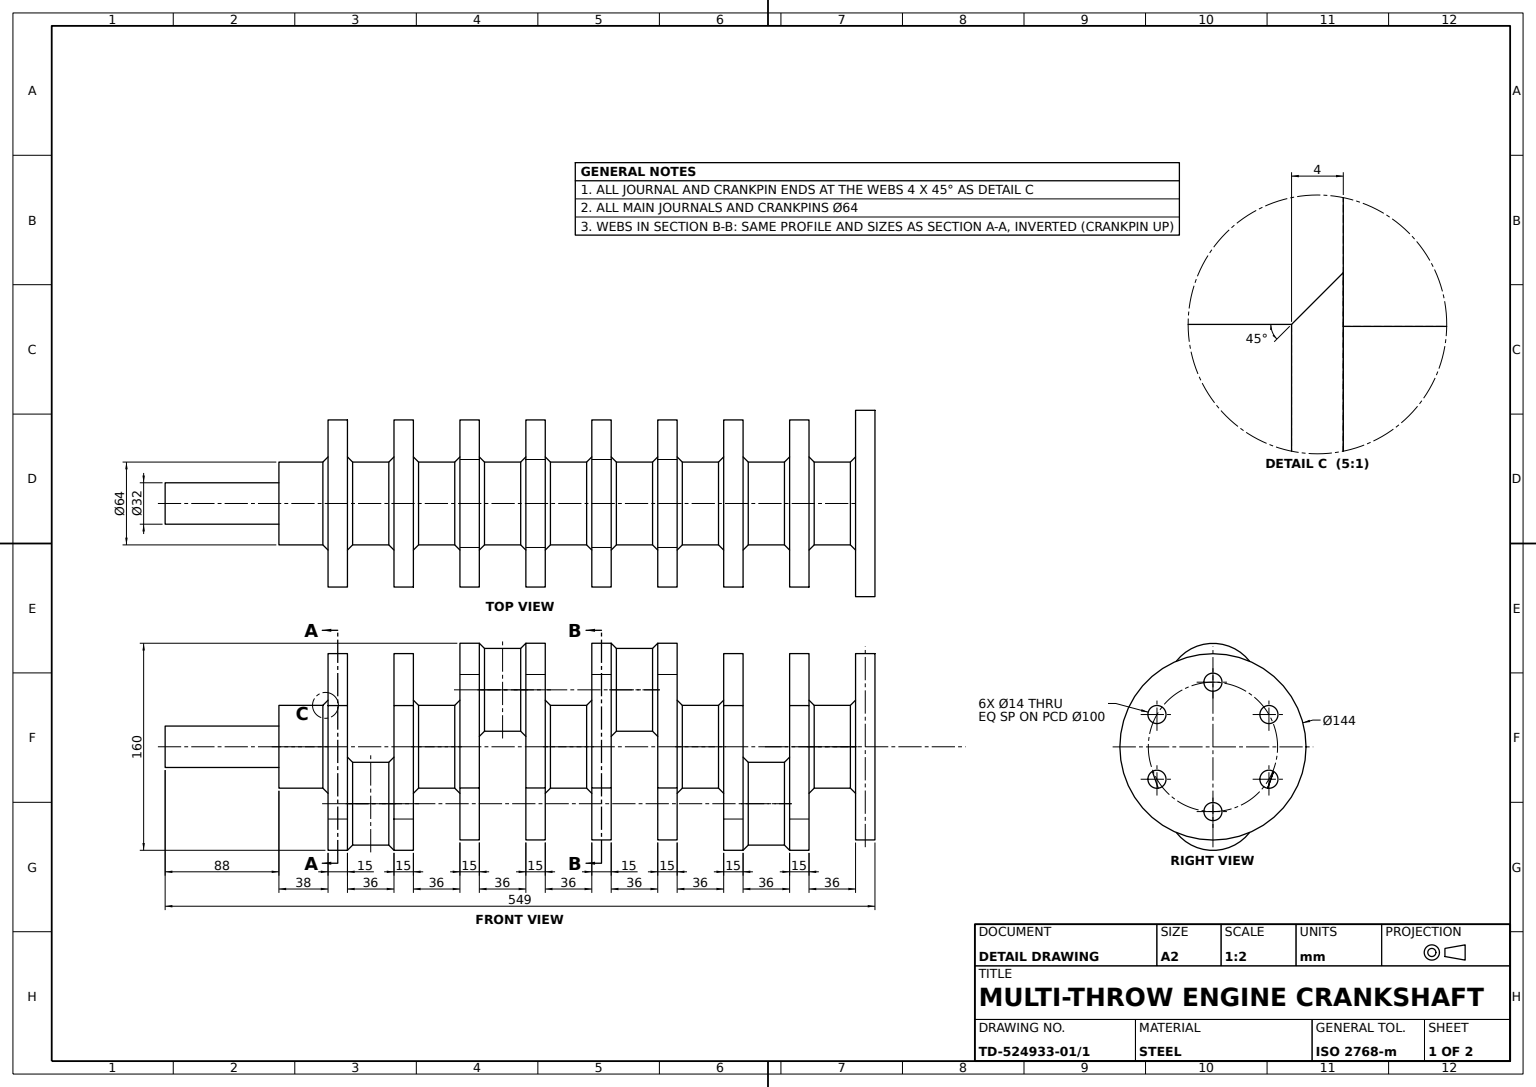
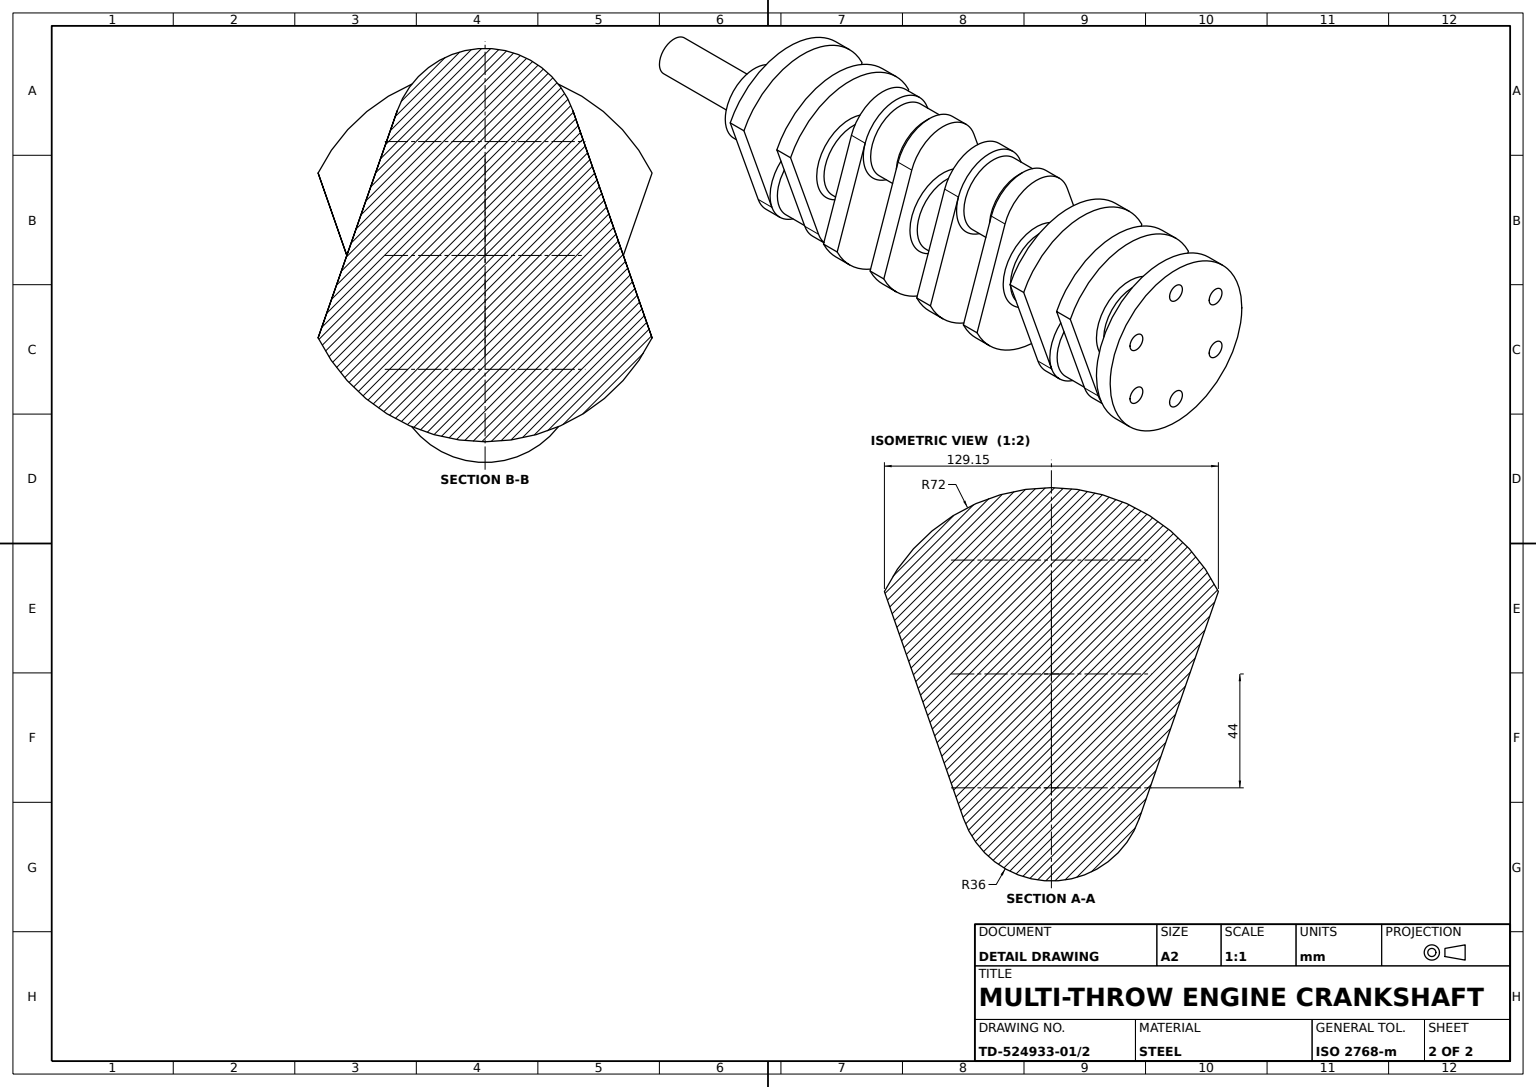
solid
v1 (32,-44,-85)
v2 (36,-44,-89)
e1 v1 v2 LINE
v3 (-36,-44,-89)
e2 v3 v2 CIRCLE(AX(P(0,-44,-89),D(0,0,-1),D(-1,0,0)),36)
v4 (-32,-44,-85)
e3 v4 v3 LINE
e4 v1 v4 CIRCLE(AX(P(0,-44,-85),D(0,0,1),D(-1,0,0)),32)
face CONE(AX(P(0,-44,-89),D(0,0,-1),D(-1,0,0)),36,0.785398163) [e1 -e2 -e3 -e4]
v5 (33.992546,55.853557,-206)
v6 (33.992546,55.853557,-191)
e5 v5 v6 LINE
v7 (-33.992546,55.853557,-206)
e6 v7 v5 CIRCLE(AX(P(0,44,-206),D(0,0,-1),D(-1,0,0)),36)
v8 (-33.992546,55.853557,-191)
e7 v7 v8 LINE
e8 v8 v6 CIRCLE(AX(P(0,44,-191),D(0,0,-1),D(-1,0,0)),36)
face CYL(AX(P(0,44,-206),D(0,0,1),D(1,0,0)),36) [-e5 -e6 e7 e8]
v9 (32,-44,-363)
v10 (-32,-44,-363)
e9 v9 v10 CIRCLE(AX(P(0,-44,-363),D(0,0,-1),D(-1,0,0)),32)
v11 (-32,-44,-391)
e10 v11 v10 LINE
v12 (32,-44,-391)
e11 v11 v12 CIRCLE(AX(P(0,-44,-391),D(0,0,1),D(-1,0,0)),32)
e12 v12 v9 LINE
face CYL(AX(P(0,-44,-395),D(0,0,1),D(1,0,0)),32) [e9 -e10 e11 e12]
v13 (-16,0,88)
v14 (16,0,88)
e13 v13 v14 CIRCLE(AX(P(0,0,88),D(0,0,1),D(1,0,0)),16)
v15 (-16,0,0)
e14 v13 v15 LINE
v16 (16,0,0)
e15 v15 v16 CIRCLE(AX(P(0,0,0),D(0,0,1),D(1,0,0)),16)
e16 v14 v16 LINE
face CYL(AX(P(0,0,88),D(0,0,-1),D(-1,0,0)),16) [-e13 e14 e15 -e16]
v17 (64.574275,-31.845926,-206)
e17 v17 v5 LINE
v18 (-64.574275,-31.845926,-206)
e18 v17 v18 CIRCLE(AX(P(0,0,-206),D(0,0,-1),D(-1,0,0)),72)
e19 v7 v18 LINE
v19 (-36,0,-206)
v20 (36,0,-206)
e20 v19 v20 CIRCLE(AX(P(0,0,-206),D(0,0,1),D(-1,0,0)),36)
e21 v20 v19 CIRCLE(AX(P(0,0,-206),D(0,0,1),D(-1,0,0)),36)
face PLANE(AX(P(0,0,-206),D(0,0,-1),D(-1,0,0))) [-e17 e18 -e19 e6] [e20 e21]
v21 (-33.992546,55.853557,-308)
v22 (-33.992546,55.853557,-293)
e22 v21 v22 LINE
v23 (-64.574275,-31.845926,-308)
e23 v21 v23 LINE
v24 (-64.574275,-31.845926,-293)
e24 v23 v24 LINE
e25 v22 v24 LINE
face PLANE(AX(P(-33.992546,55.853557,-308),D(-0.944237388,0.329265479,0),D(-0.329265479,-0.944237388,0))) [-e22 e23 e24 -e25]
v25 (36,0,-308)
v26 (-36,0,-308)
e26 v25 v26 CIRCLE(AX(P(0,0,-308),D(0,0,1),D(-1,0,0)),36)
e27 v26 v25 CIRCLE(AX(P(0,0,-308),D(0,0,1),D(-1,0,0)),36)
v27 (64.574275,-31.845926,-308)
e28 v27 v23 CIRCLE(AX(P(0,0,-308),D(0,0,-1),D(-1,0,0)),72)
v28 (33.992546,55.853557,-308)
e29 v21 v28 CIRCLE(AX(P(0,44,-308),D(0,0,-1),D(-1,0,0)),36)
e30 v27 v28 LINE
face PLANE(AX(P(0,0,-308),D(0,0,-1),D(-1,0,0))) [e26 e27] [e28 -e23 e29 -e30]
v29 (7,-50,-461)
v30 (7,-50,-446)
e31 v29 v30 LINE
v31 (-7,-50,-461)
e32 v29 v31 CIRCLE(AX(P(0,-50,-461),D(0,0,-1),D(-1,0,0)),7)
v32 (-7,-50,-446)
e33 v31 v32 LINE
e34 v30 v32 CIRCLE(AX(P(0,-50,-446),D(0,0,-1),D(-1,0,0)),7)
face CYL(AX(P(0,-50,-461),D(0,0,1),D(1,0,0)),7) rev [-e31 e32 e33 -e34]
v33 (32,0,-108)
v34 (-32,0,-108)
e35 v33 v34 CIRCLE(AX(P(0,0,-108),D(0,0,-1),D(-1,0,0)),32)
v35 (-32,0,-136)
e36 v35 v34 LINE
v36 (32,0,-136)
e37 v35 v36 CIRCLE(AX(P(0,0,-136),D(0,0,1),D(-1,0,0)),32)
e38 v36 v33 LINE
face CYL(AX(P(0,0,-140),D(0,0,1),D(1,0,0)),32) [e35 -e36 e37 e38]
v37 (36.30127,25,-461)
v38 (36.30127,25,-446)
e39 v37 v38 LINE
v39 (50.30127,25,-461)
e40 v37 v39 CIRCLE(AX(P(43.30127,25,-461),D(0,0,-1),D(-1,0,0)),7)
v40 (50.30127,25,-446)
e41 v39 v40 LINE
e42 v38 v40 CIRCLE(AX(P(43.30127,25,-446),D(0,0,-1),D(-1,0,0)),7)
face CYL(AX(P(43.30127,25,-461),D(0,0,1),D(1,0,0)),7) rev [-e39 e40 e41 -e42]
v41 (36,0,-242)
v42 (-36,0,-242)
e43 v41 v42 CIRCLE(AX(P(0,0,-242),D(0,0,-1),D(-1,0,0)),36)
e44 v42 v41 CIRCLE(AX(P(0,0,-242),D(0,0,-1),D(-1,0,0)),36)
v43 (-33.992546,55.853557,-242)
v44 (33.992546,55.853557,-242)
e45 v43 v44 CIRCLE(AX(P(0,44,-242),D(0,0,-1),D(-1,0,0)),36)
v45 (-64.574275,-31.845926,-242)
e46 v43 v45 LINE
v46 (64.574275,-31.845926,-242)
e47 v46 v45 CIRCLE(AX(P(0,0,-242),D(0,0,-1),D(-1,0,0)),72)
e48 v46 v44 LINE
face PLANE(AX(P(0,0,-242),D(0,0,-1),D(-1,0,0))) rev [e43 e44] [-e45 e46 -e47 e48]
v47 (33.992546,-55.853557,-359)
v48 (64.574275,31.845926,-359)
e49 v47 v48 LINE
v49 (36,-44,-359)
e50 v47 v49 CIRCLE(AX(P(0,-44,-359),D(0,0,1),D(-1,0,0)),36)
v50 (-36,-44,-359)
e51 v49 v50 CIRCLE(AX(P(0,-44,-359),D(0,0,1),D(-1,0,0)),36)
v51 (-33.992546,-55.853557,-359)
e52 v50 v51 CIRCLE(AX(P(0,-44,-359),D(0,0,1),D(-1,0,0)),36)
v52 (-64.574275,31.845926,-359)
e53 v52 v51 LINE
e54 v52 v48 CIRCLE(AX(P(0,0,-359),D(0,0,-1),D(-1,0,0)),72)
face PLANE(AX(P(0,0,-359),D(0,0,-1),D(-1,0,0))) [-e49 e50 e51 e52 -e53 e54]
v53 (-33.992546,-55.853557,-53)
v54 (-33.992546,-55.853557,-38)
e55 v53 v54 LINE
v55 (-64.574275,31.845926,-38)
e56 v54 v55 LINE
v56 (-64.574275,31.845926,-53)
e57 v56 v55 LINE
e58 v53 v56 LINE
face PLANE(AX(P(-64.574275,31.845926,-53),D(0.944237388,0.329265479,0),D(-0.329265479,0.944237388,0))) rev [e55 e56 -e57 -e58]
v57 (-64.574275,31.845926,-344)
e59 v52 v57 LINE
v58 (64.574275,31.845926,-344)
e60 v57 v58 CIRCLE(AX(P(0,0,-344),D(0,0,-1),D(-1,0,0)),72)
e61 v48 v58 LINE
face CYL(AX(P(0,0,-359),D(0,0,1),D(1,0,0)),72) [e59 e60 -e61 -e54]
v59 (-33.992546,-55.853557,-410)
v60 (-33.992546,-55.853557,-395)
e62 v59 v60 LINE
v61 (33.992546,-55.853557,-410)
e63 v61 v59 CIRCLE(AX(P(0,-44,-410),D(0,0,-1),D(-1,0,0)),36)
v62 (33.992546,-55.853557,-395)
e64 v61 v62 LINE
e65 v62 v60 CIRCLE(AX(P(0,-44,-395),D(0,0,-1),D(-1,0,0)),36)
face CYL(AX(P(0,-44,-410),D(0,0,1),D(1,0,0)),36) [-e62 -e63 e64 e65]
v63 (36,0,-410)
v64 (-36,0,-410)
e66 v63 v64 CIRCLE(AX(P(0,0,-410),D(0,0,1),D(-1,0,0)),36)
v65 (32,0,-414)
e67 v65 v63 LINE
v66 (-32,0,-414)
e68 v66 v65 CIRCLE(AX(P(0,0,-414),D(0,0,-1),D(-1,0,0)),32)
e69 v66 v64 LINE
face CONE(AX(P(0,0,-414),D(0,0,1),D(1,0,0)),32,0.785398163) [-e66 -e67 -e68 e69]
v67 (33.992546,55.853557,-155)
v68 (64.574275,-31.845926,-155)
e70 v67 v68 LINE
v69 (33.992546,55.853557,-140)
e71 v67 v69 LINE
v70 (64.574275,-31.845926,-140)
e72 v69 v70 LINE
e73 v68 v70 LINE
face PLANE(AX(P(64.574275,-31.845926,-155),D(-0.944237388,-0.329265479,0),D(0.329265479,-0.944237388,0))) rev [-e70 e71 e72 -e73]
v71 (-33.992546,55.853557,-140)
e74 v71 v69 CIRCLE(AX(P(0,44,-140),D(0,0,-1),D(-1,0,0)),36)
v72 (-64.574275,-31.845926,-140)
e75 v72 v71 LINE
e76 v70 v72 CIRCLE(AX(P(0,0,-140),D(0,0,-1),D(-1,0,0)),72)
v73 (-36,0,-140)
v74 (36,0,-140)
e77 v73 v74 CIRCLE(AX(P(0,0,-140),D(0,0,-1),D(-1,0,0)),36)
e78 v74 v73 CIRCLE(AX(P(0,0,-140),D(0,0,-1),D(-1,0,0)),36)
face PLANE(AX(P(0,0,-140),D(0,0,-1),D(-1,0,0))) rev [-e72 -e74 -e75 -e76] [e77 e78]
v75 (50.30127,-25,-461)
v76 (36.30127,-25,-461)
e79 v75 v76 CIRCLE(AX(P(43.30127,-25,-461),D(0,0,-1),D(-1,0,0)),7)
v77 (36.30127,-25,-446)
e80 v76 v77 LINE
v78 (50.30127,-25,-446)
e81 v78 v77 CIRCLE(AX(P(43.30127,-25,-446),D(0,0,-1),D(-1,0,0)),7)
e82 v75 v78 LINE
face CYL(AX(P(43.30127,-25,-461),D(0,0,1),D(1,0,0)),7) rev [e79 e80 -e81 -e82]
v79 (-32,0,-312)
e83 v79 v26 LINE
v80 (32,0,-312)
e84 v80 v79 CIRCLE(AX(P(0,0,-312),D(0,0,-1),D(-1,0,0)),32)
e85 v80 v25 LINE
face CONE(AX(P(0,0,-312),D(0,0,1),D(1,0,0)),32,0.785398163) [-e83 -e84 e85 -e27]
v81 (33.992546,55.853557,-293)
e86 v22 v81 CIRCLE(AX(P(0,44,-293),D(0,0,-1),D(-1,0,0)),36)
e87 v28 v81 LINE
face CYL(AX(P(0,44,-308),D(0,0,1),D(1,0,0)),36) [e22 e86 -e87 -e29]
e88 v9 v49 LINE
e89 v10 v9 CIRCLE(AX(P(0,-44,-363),D(0,0,-1),D(-1,0,0)),32)
e90 v10 v50 LINE
face CONE(AX(P(0,-44,-363),D(0,0,1),D(1,0,0)),32,0.785398163) [-e88 -e89 e90 -e51]
v82 (-32,44,-261)
v83 (-36,44,-257)
e91 v82 v83 LINE
v84 (32,44,-261)
e92 v84 v82 CIRCLE(AX(P(0,44,-261),D(0,0,-1),D(-1,0,0)),32)
v85 (36,44,-257)
e93 v84 v85 LINE
e94 v83 v85 CIRCLE(AX(P(0,44,-257),D(0,0,1),D(-1,0,0)),36)
face CONE(AX(P(0,44,-261),D(0,0,1),D(1,0,0)),32,0.785398163) [-e91 -e92 e93 -e94]
v86 (-33.992546,55.853557,-155)
e95 v86 v67 CIRCLE(AX(P(0,44,-155),D(0,0,-1),D(-1,0,0)),36)
e96 v86 v71 LINE
face CYL(AX(P(0,44,-155),D(0,0,1),D(1,0,0)),36) [e74 -e71 -e95 e96]
v87 (72,0,-461)
v88 (72,0,-446)
e97 v87 v88 LINE
v89 (-72,0,-461)
e98 v89 v87 CIRCLE(AX(P(0,0,-461),D(0,0,-1),D(-1,0,0)),72)
v90 (-72,0,-446)
e99 v89 v90 LINE
e100 v90 v88 CIRCLE(AX(P(0,0,-446),D(0,0,-1),D(-1,0,0)),72)
face CYL(AX(P(0,0,-461),D(0,0,1),D(1,0,0)),72) [-e97 -e98 e99 e100]
v91 (-32,0,-442)
e101 v91 v66 LINE
v92 (32,0,-442)
e102 v91 v92 CIRCLE(AX(P(0,0,-442),D(0,0,1),D(-1,0,0)),32)
e103 v92 v65 LINE
e104 v65 v66 CIRCLE(AX(P(0,0,-414),D(0,0,-1),D(-1,0,0)),32)
face CYL(AX(P(0,0,-446),D(0,0,1),D(1,0,0)),32) [-e101 e102 e103 e104]
e105 v92 v91 CIRCLE(AX(P(0,0,-442),D(0,0,1),D(-1,0,0)),32)
face CYL(AX(P(0,0,-446),D(0,0,1),D(1,0,0)),32) [e101 e68 -e103 e105]
e106 v88 v90 CIRCLE(AX(P(0,0,-446),D(0,0,-1),D(-1,0,0)),72)
e107 v87 v89 CIRCLE(AX(P(0,0,-461),D(0,0,-1),D(-1,0,0)),72)
face CYL(AX(P(0,0,-461),D(0,0,1),D(1,0,0)),72) [e106 -e99 -e107 e97]
e108 v64 v63 CIRCLE(AX(P(0,0,-410),D(0,0,1),D(-1,0,0)),36)
face CONE(AX(P(0,0,-414),D(0,0,1),D(1,0,0)),32,0.785398163) [-e108 -e69 -e104 e67]
v93 (32,0,-34)
v94 (32,0,0)
e109 v93 v94 LINE
v95 (-32,0,-34)
e110 v93 v95 CIRCLE(AX(P(0,0,-34),D(0,0,1),D(-1,0,0)),32)
v96 (-32,0,0)
e111 v95 v96 LINE
e112 v96 v94 CIRCLE(AX(P(0,0,0),D(0,0,-1),D(-1,0,0)),32)
face CYL(AX(P(0,0,-38),D(0,0,1),D(1,0,0)),32) [-e109 e110 e111 e112]
v97 (64.574275,-31.845926,-191)
v98 (-64.574275,-31.845926,-191)
e113 v97 v98 CIRCLE(AX(P(0,0,-191),D(0,0,-1),D(-1,0,0)),72)
e114 v97 v6 LINE
v99 (36,44,-191)
e115 v6 v99 CIRCLE(AX(P(0,44,-191),D(0,0,-1),D(-1,0,0)),36)
v100 (-36,44,-191)
e116 v99 v100 CIRCLE(AX(P(0,44,-191),D(0,0,-1),D(-1,0,0)),36)
e117 v100 v8 CIRCLE(AX(P(0,44,-191),D(0,0,-1),D(-1,0,0)),36)
e118 v8 v98 LINE
face PLANE(AX(P(0,0,-191),D(0,0,-1),D(-1,0,0))) rev [-e113 e114 e115 e116 e117 e118]
v101 (-36,-44,-395)
e119 v11 v101 LINE
e120 v60 v101 CIRCLE(AX(P(0,-44,-395),D(0,0,-1),D(-1,0,0)),36)
v102 (36,-44,-395)
e121 v102 v62 CIRCLE(AX(P(0,-44,-395),D(0,0,-1),D(-1,0,0)),36)
e122 v12 v102 LINE
face CONE(AX(P(0,-44,-395),D(0,0,-1),D(-1,0,0)),36,0.785398163) [e119 -e120 -e65 -e121 -e122 -e11]
v103 (-64.574275,31.845926,-410)
v104 (-64.574275,31.845926,-395)
e123 v103 v104 LINE
e124 v103 v59 LINE
e125 v104 v60 LINE
face PLANE(AX(P(-33.992546,-55.853557,-410),D(-0.944237388,-0.329265479,0),D(0.329265479,-0.944237388,0))) [-e123 e124 e62 -e125]
v105 (-36,0,-104)
e126 v34 v105 LINE
v106 (36,0,-104)
e127 v106 v105 CIRCLE(AX(P(0,0,-104),D(0,0,1),D(-1,0,0)),36)
e128 v33 v106 LINE
e129 v34 v33 CIRCLE(AX(P(0,0,-108),D(0,0,-1),D(-1,0,0)),32)
face CONE(AX(P(0,0,-108),D(0,0,1),D(1,0,0)),32,0.785398163) [e126 -e127 -e128 -e129]
v107 (-36.30127,25,-446)
v108 (-50.30127,25,-446)
e130 v107 v108 CIRCLE(AX(P(-43.30127,25,-446),D(0,0,-1),D(-1,0,0)),7)
e131 v108 v107 CIRCLE(AX(P(-43.30127,25,-446),D(0,0,-1),D(-1,0,0)),7)
v109 (-7,50,-446)
v110 (7,50,-446)
e132 v109 v110 CIRCLE(AX(P(0,50,-446),D(0,0,-1),D(-1,0,0)),7)
e133 v110 v109 CIRCLE(AX(P(0,50,-446),D(0,0,-1),D(-1,0,0)),7)
e134 v40 v38 CIRCLE(AX(P(43.30127,25,-446),D(0,0,-1),D(-1,0,0)),7)
e135 v77 v78 CIRCLE(AX(P(43.30127,-25,-446),D(0,0,-1),D(-1,0,0)),7)
e136 v32 v30 CIRCLE(AX(P(0,-50,-446),D(0,0,-1),D(-1,0,0)),7)
v111 (36,0,-446)
v112 (-36,0,-446)
e137 v111 v112 CIRCLE(AX(P(0,0,-446),D(0,0,-1),D(-1,0,0)),36)
e138 v112 v111 CIRCLE(AX(P(0,0,-446),D(0,0,-1),D(-1,0,0)),36)
v113 (-36.30127,-25,-446)
v114 (-50.30127,-25,-446)
e139 v113 v114 CIRCLE(AX(P(-43.30127,-25,-446),D(0,0,-1),D(-1,0,0)),7)
e140 v114 v113 CIRCLE(AX(P(-43.30127,-25,-446),D(0,0,-1),D(-1,0,0)),7)
face PLANE(AX(P(0,0,-446),D(0,0,-1),D(-1,0,0))) rev [e130 e131] [e132 e133] [e134 e42] [e81 e135] [-e100 -e106] [e136 e34] [e137 e138] [e139 e140]
v115 (-36,0,-344)
v116 (36,0,-344)
e141 v115 v116 CIRCLE(AX(P(0,0,-344),D(0,0,-1),D(-1,0,0)),36)
v117 (-32,0,-340)
e142 v117 v115 LINE
v118 (32,0,-340)
e143 v118 v117 CIRCLE(AX(P(0,0,-340),D(0,0,1),D(-1,0,0)),32)
e144 v118 v116 LINE
face CONE(AX(P(0,0,-344),D(0,0,-1),D(-1,0,0)),36,0.785398163) [-e141 -e142 -e143 e144]
e145 v36 v74 LINE
e146 v35 v73 LINE
face CONE(AX(P(0,0,-140),D(0,0,-1),D(-1,0,0)),36,0.785398163) [-e145 -e37 e146 -e78]
e147 v79 v80 CIRCLE(AX(P(0,0,-312),D(0,0,-1),D(-1,0,0)),32)
e148 v118 v80 LINE
e149 v117 v79 LINE
face CYL(AX(P(0,0,-344),D(0,0,1),D(1,0,0)),32) [e147 -e148 e143 e149]
e150 v117 v118 CIRCLE(AX(P(0,0,-340),D(0,0,1),D(-1,0,0)),32)
e151 v116 v115 CIRCLE(AX(P(0,0,-344),D(0,0,-1),D(-1,0,0)),36)
face CONE(AX(P(0,0,-344),D(0,0,-1),D(-1,0,0)),36,0.785398163) [-e150 e142 -e151 -e144]
v119 (-36,-44,-53)
e152 v119 v53 CIRCLE(AX(P(0,-44,-53),D(0,0,1),D(-1,0,0)),36)
v120 (64.574275,31.845926,-53)
e153 v56 v120 CIRCLE(AX(P(0,0,-53),D(0,0,-1),D(-1,0,0)),72)
v121 (33.992546,-55.853557,-53)
e154 v120 v121 LINE
v122 (36,-44,-53)
e155 v121 v122 CIRCLE(AX(P(0,-44,-53),D(0,0,1),D(-1,0,0)),36)
e156 v122 v119 CIRCLE(AX(P(0,-44,-53),D(0,0,1),D(-1,0,0)),36)
face PLANE(AX(P(0,-44,-53),D(0,0,-1),D(-1,0,0))) [e152 e58 e153 e154 e155 e156]
v123 (33.992546,-55.853557,-89)
v124 (-33.992546,-55.853557,-89)
e157 v123 v124 CIRCLE(AX(P(0,-44,-89),D(0,0,-1),D(-1,0,0)),36)
v125 (-33.992546,-55.853557,-104)
e158 v125 v124 LINE
v126 (33.992546,-55.853557,-104)
e159 v126 v125 CIRCLE(AX(P(0,-44,-104),D(0,0,-1),D(-1,0,0)),36)
e160 v126 v123 LINE
face CYL(AX(P(0,-44,-104),D(0,0,1),D(1,0,0)),36) [e157 -e158 -e159 e160]
v127 (32,0,-210)
e161 v127 v20 LINE
v128 (-32,0,-210)
e162 v128 v127 CIRCLE(AX(P(0,0,-210),D(0,0,-1),D(-1,0,0)),32)
e163 v128 v19 LINE
face CONE(AX(P(0,0,-210),D(0,0,1),D(1,0,0)),32,0.785398163) [-e161 -e162 e163 -e21]
v129 (-33.992546,-55.853557,-344)
e164 v51 v129 LINE
e165 v47 v51 CIRCLE(AX(P(0,-44,-359),D(0,0,-1),D(-1,0,0)),36)
v130 (33.992546,-55.853557,-344)
e166 v47 v130 LINE
e167 v130 v129 CIRCLE(AX(P(0,-44,-344),D(0,0,-1),D(-1,0,0)),36)
face CYL(AX(P(0,-44,-359),D(0,0,1),D(1,0,0)),36) [-e164 -e165 e166 e167]
v131 (-32,44,-159)
v132 (32,44,-159)
e168 v131 v132 CIRCLE(AX(P(0,44,-159),D(0,0,-1),D(-1,0,0)),32)
v133 (32,44,-187)
e169 v133 v132 LINE
v134 (-32,44,-187)
e170 v133 v134 CIRCLE(AX(P(0,44,-187),D(0,0,1),D(-1,0,0)),32)
e171 v134 v131 LINE
face CYL(AX(P(0,44,-191),D(0,0,1),D(1,0,0)),32) [e168 -e169 e170 e171]
v135 (32,0,-238)
e172 v135 v127 LINE
v136 (-32,0,-238)
e173 v135 v136 CIRCLE(AX(P(0,0,-238),D(0,0,1),D(-1,0,0)),32)
e174 v136 v128 LINE
face CYL(AX(P(0,0,-242),D(0,0,1),D(1,0,0)),32) [-e172 e173 e174 e162]
e175 v134 v100 LINE
e176 v133 v99 LINE
face CONE(AX(P(0,44,-191),D(0,0,-1),D(-1,0,0)),36,0.785398163) [-e115 -e8 -e117 -e175 -e170 e176]
v137 (64.574275,31.845926,-38)
v138 (33.992546,-55.853557,-38)
e177 v137 v138 LINE
e178 v121 v138 LINE
e179 v120 v137 LINE
face PLANE(AX(P(64.574275,31.845926,-53),D(-0.944237388,0.329265479,0),D(-0.329265479,-0.944237388,0))) rev [e177 -e178 -e154 e179]
v139 (-64.574275,-31.845926,-155)
e180 v139 v72 LINE
e181 v68 v139 CIRCLE(AX(P(0,0,-155),D(0,0,-1),D(-1,0,0)),72)
face CYL(AX(P(0,0,-155),D(0,0,1),D(1,0,0)),72) [e73 e76 -e180 -e181]
v140 (32,44,-289)
v141 (36,44,-293)
e182 v140 v141 LINE
e183 v81 v141 CIRCLE(AX(P(0,44,-293),D(0,0,-1),D(-1,0,0)),36)
v142 (-36,44,-293)
e184 v142 v22 CIRCLE(AX(P(0,44,-293),D(0,0,-1),D(-1,0,0)),36)
v143 (-32,44,-289)
e185 v143 v142 LINE
e186 v140 v143 CIRCLE(AX(P(0,44,-289),D(0,0,1),D(-1,0,0)),32)
face CONE(AX(P(0,44,-293),D(0,0,-1),D(-1,0,0)),36,0.785398163) [e182 -e183 -e86 -e184 -e185 -e186]
v144 (32,-44,-57)
e187 v1 v144 LINE
v145 (-32,-44,-57)
e188 v4 v145 LINE
e189 v145 v144 CIRCLE(AX(P(0,-44,-57),D(0,0,-1),D(-1,0,0)),32)
face CYL(AX(P(0,-44,-89),D(0,0,1),D(1,0,0)),32) [-e187 e4 e188 e189]
e190 v92 v111 LINE
e191 v91 v112 LINE
face CONE(AX(P(0,0,-446),D(0,0,-1),D(-1,0,0)),36,0.785398163) [-e137 -e190 -e102 e191]
e192 v31 v29 CIRCLE(AX(P(0,-50,-461),D(0,0,-1),D(-1,0,0)),7)
face CYL(AX(P(0,-50,-461),D(0,0,1),D(1,0,0)),7) rev [e31 -e136 -e33 e192]
e193 v143 v82 LINE
e194 v82 v84 CIRCLE(AX(P(0,44,-261),D(0,0,-1),D(-1,0,0)),32)
e195 v140 v84 LINE
face CYL(AX(P(0,44,-293),D(0,0,1),D(1,0,0)),32) [e193 e194 -e195 e186]
e196 v134 v133 CIRCLE(AX(P(0,44,-187),D(0,0,1),D(-1,0,0)),32)
face CONE(AX(P(0,44,-191),D(0,0,-1),D(-1,0,0)),36,0.785398163) [-e176 -e196 e175 -e116]
e197 v18 v98 LINE
face PLANE(AX(P(-33.992546,55.853557,-206),D(-0.944237388,0.329265479,0),D(-0.329265479,-0.944237388,0))) [e19 e197 -e118 -e7]
v146 (-64.574275,-31.845926,-257)
e198 v146 v45 LINE
v147 (64.574275,-31.845926,-257)
e199 v147 v146 CIRCLE(AX(P(0,0,-257),D(0,0,-1),D(-1,0,0)),72)
e200 v147 v46 LINE
face CYL(AX(P(0,0,-257),D(0,0,1),D(1,0,0)),72) [e47 -e198 -e199 e200]
e201 v36 v35 CIRCLE(AX(P(0,0,-136),D(0,0,1),D(-1,0,0)),32)
face CONE(AX(P(0,0,-140),D(0,0,-1),D(-1,0,0)),36,0.785398163) [-e201 e145 -e77 -e146]
face CYL(AX(P(0,0,-344),D(0,0,1),D(1,0,0)),32) [-e149 e150 e148 e84]
e202 v144 v145 CIRCLE(AX(P(0,-44,-57),D(0,0,-1),D(-1,0,0)),32)
e203 v4 v1 CIRCLE(AX(P(0,-44,-85),D(0,0,1),D(-1,0,0)),32)
face CYL(AX(P(0,-44,-89),D(0,0,1),D(1,0,0)),32) [e202 -e188 e203 e187]
e204 v17 v97 LINE
face PLANE(AX(P(33.992546,55.853557,-206),D(0.944237388,0.329265479,0),D(-0.329265479,0.944237388,0))) [-e114 -e204 e17 e5]
e205 v136 v135 CIRCLE(AX(P(0,0,-238),D(0,0,1),D(-1,0,0)),32)
e206 v127 v128 CIRCLE(AX(P(0,0,-210),D(0,0,-1),D(-1,0,0)),32)
face CYL(AX(P(0,0,-242),D(0,0,1),D(1,0,0)),32) [e205 e172 e206 -e174]
e207 v130 v58 LINE
e208 v57 v129 LINE
face PLANE(AX(P(0,0,-344),D(0,0,-1),D(-1,0,0))) rev [e141 e151] [e207 -e60 e208 -e167]
e209 v14 v13 CIRCLE(AX(P(0,0,88),D(0,0,1),D(1,0,0)),16)
face PLANE(AX(P(0,0,88),D(0,0,1),D(1,0,0))) [e13 e209]
e210 v143 v140 CIRCLE(AX(P(0,44,-289),D(0,0,1),D(-1,0,0)),32)
e211 v141 v142 CIRCLE(AX(P(0,44,-293),D(0,0,-1),D(-1,0,0)),36)
face CONE(AX(P(0,44,-293),D(0,0,-1),D(-1,0,0)),36,0.785398163) [-e210 e185 -e211 -e182]
v148 (-50.30127,25,-461)
e212 v148 v108 LINE
v149 (-36.30127,25,-461)
e213 v148 v149 CIRCLE(AX(P(-43.30127,25,-461),D(0,0,-1),D(-1,0,0)),7)
e214 v149 v107 LINE
face CYL(AX(P(-43.30127,25,-461),D(0,0,1),D(1,0,0)),7) rev [-e212 e213 e214 -e131]
face CYL(AX(P(0,0,-206),D(0,0,1),D(1,0,0)),72) [-e197 -e18 e204 e113]
face CONE(AX(P(0,0,-210),D(0,0,1),D(1,0,0)),32,0.785398163) [e161 -e20 -e163 -e206]
face PLANE(AX(P(47.672356,-16.62385,-359),D(0.944237388,-0.329265479,0),D(0.329265479,0.944237388,0))) [-e166 e49 e61 -e207]
v150 (-64.574275,31.845926,-104)
v151 (-64.574275,31.845926,-89)
e215 v150 v151 LINE
e216 v150 v125 LINE
e217 v151 v124 LINE
face PLANE(AX(P(-33.992546,-55.853557,-104),D(-0.944237388,-0.329265479,0),D(0.329265479,-0.944237388,0))) [-e215 e216 e158 -e217]
e218 v132 v131 CIRCLE(AX(P(0,44,-159),D(0,0,-1),D(-1,0,0)),32)
v152 (36,44,-155)
e219 v132 v152 LINE
v153 (-36,44,-155)
e220 v153 v152 CIRCLE(AX(P(0,44,-155),D(0,0,1),D(-1,0,0)),36)
e221 v131 v153 LINE
face CONE(AX(P(0,44,-159),D(0,0,1),D(1,0,0)),32,0.785398163) [-e218 e219 -e220 -e221]
v154 (64.574275,31.845926,-395)
e222 v62 v154 LINE
e223 v104 v154 CIRCLE(AX(P(0,0,-395),D(0,0,-1),D(-1,0,0)),72)
e224 v101 v102 CIRCLE(AX(P(0,-44,-395),D(0,0,-1),D(-1,0,0)),36)
face PLANE(AX(P(0,0,-395),D(0,0,-1),D(-1,0,0))) rev [e121 e222 -e223 e125 e120 e224]
e225 v138 v54 CIRCLE(AX(P(0,-44,-38),D(0,0,-1),D(-1,0,0)),36)
e226 v121 v53 CIRCLE(AX(P(0,-44,-53),D(0,0,-1),D(-1,0,0)),36)
face CYL(AX(P(0,-44,-53),D(0,0,1),D(1,0,0)),36) [e178 e225 -e55 -e226]
e227 v144 v122 LINE
e228 v145 v119 LINE
face CONE(AX(P(0,-44,-57),D(0,0,1),D(1,0,0)),32,0.785398163) [-e156 -e227 -e189 e228]
face CYL(AX(P(0,44,-293),D(0,0,1),D(1,0,0)),32) [-e193 e210 e195 e92]
v155 (64.574275,31.845926,-410)
e229 v103 v155 CIRCLE(AX(P(0,0,-410),D(0,0,-1),D(-1,0,0)),72)
e230 v61 v155 LINE
face PLANE(AX(P(0,0,-410),D(0,0,-1),D(-1,0,0))) [e108 e66] [e229 -e230 e63 -e124]
e231 v135 v41 LINE
e232 v136 v42 LINE
face CONE(AX(P(0,0,-242),D(0,0,-1),D(-1,0,0)),36,0.785398163) [e231 -e44 -e232 -e173]
v156 (7,50,-461)
e233 v156 v110 LINE
v157 (-7,50,-461)
e234 v156 v157 CIRCLE(AX(P(0,50,-461),D(0,0,-1),D(-1,0,0)),7)
e235 v157 v109 LINE
face CYL(AX(P(0,50,-461),D(0,0,1),D(1,0,0)),7) rev [-e233 e234 e235 -e133]
v158 (64.574275,-31.845926,-293)
e236 v158 v24 CIRCLE(AX(P(0,0,-293),D(0,0,-1),D(-1,0,0)),72)
e237 v27 v158 LINE
face CYL(AX(P(0,0,-308),D(0,0,1),D(1,0,0)),72) [e236 -e24 -e28 e237]
v159 (64.574275,31.845926,-104)
e238 v150 v159 CIRCLE(AX(P(0,0,-104),D(0,0,-1),D(-1,0,0)),72)
v160 (64.574275,31.845926,-89)
e239 v151 v160 CIRCLE(AX(P(0,0,-89),D(0,0,-1),D(-1,0,0)),72)
e240 v159 v160 LINE
face CYL(AX(P(0,0,-104),D(0,0,1),D(1,0,0)),72) [-e238 e215 e239 -e240]
e241 v124 v3 CIRCLE(AX(P(0,-44,-89),D(0,0,-1),D(-1,0,0)),36)
e242 v2 v123 CIRCLE(AX(P(0,-44,-89),D(0,0,-1),D(-1,0,0)),36)
e243 v123 v160 LINE
face PLANE(AX(P(0,0,-89),D(0,0,-1),D(-1,0,0))) rev [-e239 e217 e241 e2 e242 e243]
face CYL(AX(P(0,0,-140),D(0,0,1),D(1,0,0)),32) [e201 e36 e129 -e38]
e244 v39 v37 CIRCLE(AX(P(43.30127,25,-461),D(0,0,-1),D(-1,0,0)),7)
face CYL(AX(P(43.30127,25,-461),D(0,0,1),D(1,0,0)),7) rev [-e41 e244 e39 -e134]
e245 v139 v86 LINE
face PLANE(AX(P(-64.574275,-31.845926,-155),D(0.944237388,-0.329265479,0),D(0.329265479,0.944237388,0))) rev [e75 -e96 -e245 e180]
e246 v158 v81 LINE
face PLANE(AX(P(0,0,-293),D(0,0,-1),D(-1,0,0))) rev [e25 -e236 e246 e183 e211 e184]
e247 v149 v148 CIRCLE(AX(P(-43.30127,25,-461),D(0,0,-1),D(-1,0,0)),7)
face CYL(AX(P(-43.30127,25,-461),D(0,0,1),D(1,0,0)),7) rev [-e214 e247 e212 -e130]
v161 (33.992546,55.853557,-257)
e248 v147 v161 LINE
v162 (-33.992546,55.853557,-257)
e249 v162 v146 LINE
e250 v162 v83 CIRCLE(AX(P(0,44,-257),D(0,0,1),D(-1,0,0)),36)
e251 v85 v161 CIRCLE(AX(P(0,44,-257),D(0,0,1),D(-1,0,0)),36)
face PLANE(AX(P(0,0,-257),D(0,0,-1),D(-1,0,0))) [-e248 e199 -e249 e250 e94 e251]
e252 v157 v156 CIRCLE(AX(P(0,50,-461),D(0,0,-1),D(-1,0,0)),7)
e253 v76 v75 CIRCLE(AX(P(43.30127,-25,-461),D(0,0,-1),D(-1,0,0)),7)
v163 (-36.30127,-25,-461)
v164 (-50.30127,-25,-461)
e254 v163 v164 CIRCLE(AX(P(-43.30127,-25,-461),D(0,0,-1),D(-1,0,0)),7)
e255 v164 v163 CIRCLE(AX(P(-43.30127,-25,-461),D(0,0,-1),D(-1,0,0)),7)
face PLANE(AX(P(0,0,-461),D(0,0,-1),D(-1,0,0))) [-e213 -e247] [-e192 -e32] [-e244 -e40] [-e234 -e252] [-e79 -e253] [e98 e107] [-e254 -e255]
e256 v126 v159 LINE
face PLANE(AX(P(33.992546,-55.853557,-104),D(0.944237388,-0.329265479,0),D(0.329265479,0.944237388,0))) [e240 -e243 -e160 e256]
face CONE(AX(P(0,-44,-57),D(0,0,1),D(1,0,0)),32,0.785398163) [-e202 e227 -e155 e226 -e152 -e228]
face CYL(AX(P(0,50,-461),D(0,0,1),D(1,0,0)),7) rev [-e132 -e235 e252 e233]
e257 v55 v137 CIRCLE(AX(P(0,0,-38),D(0,0,-1),D(-1,0,0)),72)
face CYL(AX(P(0,0,-53),D(0,0,1),D(1,0,0)),72) [-e179 -e153 e57 e257]
e258 v152 v67 CIRCLE(AX(P(0,44,-155),D(0,0,1),D(-1,0,0)),36)
e259 v86 v153 CIRCLE(AX(P(0,44,-155),D(0,0,1),D(-1,0,0)),36)
face CONE(AX(P(0,44,-159),D(0,0,1),D(1,0,0)),32,0.785398163) [e95 -e258 -e219 -e168 e221 -e259]
e260 v162 v43 LINE
face PLANE(AX(P(-47.672356,16.62385,-257),D(-0.944237388,0.329265479,0),D(-0.329265479,-0.944237388,0))) [-e260 e249 e198 -e46]
v165 (36,0,-38)
v166 (-36,0,-38)
e261 v165 v166 CIRCLE(AX(P(0,0,-38),D(0,0,-1),D(-1,0,0)),36)
e262 v166 v165 CIRCLE(AX(P(0,0,-38),D(0,0,-1),D(-1,0,0)),36)
face PLANE(AX(P(0,-44,-38),D(0,0,-1),D(-1,0,0))) rev [e261 e262] [-e56 -e225 -e177 -e257]
face CONE(AX(P(0,-44,-363),D(0,0,1),D(1,0,0)),32,0.785398163) [-e90 -e9 e88 -e50 e165 -e52]
face PLANE(AX(P(-47.672356,-16.62385,-359),D(-0.944237388,-0.329265479,0),D(0.329265479,-0.944237388,0))) [-e59 e53 e164 -e208]
e263 v155 v154 LINE
face CYL(AX(P(0,0,-410),D(0,0,1),D(1,0,0)),72) [-e263 -e229 e123 e223]
face CONE(AX(P(0,-44,-89),D(0,0,-1),D(-1,0,0)),36,0.785398163) [e3 -e241 -e157 -e242 -e1 -e203]
face PLANE(AX(P(33.992546,-55.853557,-410),D(0.944237388,-0.329265479,0),D(0.329265479,0.944237388,0))) [-e64 e230 e263 -e222]
e264 v95 v93 CIRCLE(AX(P(0,0,-34),D(0,0,1),D(-1,0,0)),32)
e265 v95 v166 LINE
e266 v93 v165 LINE
face CONE(AX(P(0,0,-38),D(0,0,-1),D(-1,0,0)),36,0.785398163) [-e264 e265 -e261 -e266]
e267 v163 v113 LINE
e268 v164 v114 LINE
face CYL(AX(P(-43.30127,-25,-461),D(0,0,1),D(1,0,0)),7) rev [e255 e267 -e140 -e268]
face CYL(AX(P(0,44,-191),D(0,0,1),D(1,0,0)),32) [-e171 e196 e169 e218]
face CONE(AX(P(0,0,-38),D(0,0,-1),D(-1,0,0)),36,0.785398163) [e266 -e262 -e265 -e110]
face CYL(AX(P(43.30127,-25,-461),D(0,0,1),D(1,0,0)),7) rev [-e135 -e80 e253 e82]
face PLANE(AX(P(0,0,-155),D(0,0,-1),D(-1,0,0))) [e258 e70 e181 e245 e259 e220]
face CONE(AX(P(0,0,-312),D(0,0,1),D(1,0,0)),32,0.785398163) [-e147 e83 -e26 -e85]
e269 v162 v161 CIRCLE(AX(P(0,44,-257),D(0,0,-1),D(-1,0,0)),36)
face CONE(AX(P(0,44,-261),D(0,0,1),D(1,0,0)),32,0.785398163) [-e194 e91 -e250 e269 -e251 -e93]
face CYL(AX(P(-43.30127,-25,-461),D(0,0,1),D(1,0,0)),7) rev [-e267 e254 e268 -e139]
e270 v105 v106 CIRCLE(AX(P(0,0,-104),D(0,0,1),D(-1,0,0)),36)
face CONE(AX(P(0,0,-108),D(0,0,1),D(1,0,0)),32,0.785398163) [-e35 e128 -e270 -e126]
face CONE(AX(P(0,0,-446),D(0,0,-1),D(-1,0,0)),36,0.785398163) [-e138 -e191 -e105 e190]
e271 v12 v11 CIRCLE(AX(P(0,-44,-391),D(0,0,1),D(-1,0,0)),32)
face CYL(AX(P(0,-44,-395),D(0,0,1),D(1,0,0)),32) [e10 e89 -e12 e271]
e272 v161 v44 LINE
face PLANE(AX(P(47.672356,16.62385,-257),D(0.944237388,0.329265479,0),D(-0.329265479,0.944237388,0))) [e248 e272 -e48 -e200]
face CONE(AX(P(0,0,-242),D(0,0,-1),D(-1,0,0)),36,0.785398163) [e232 -e43 -e231 -e205]
face CONE(AX(P(0,-44,-395),D(0,0,-1),D(-1,0,0)),36,0.785398163) [-e271 e122 -e224 -e119]
e273 v16 v15 CIRCLE(AX(P(0,0,0),D(0,0,1),D(1,0,0)),16)
face CYL(AX(P(0,0,88),D(0,0,-1),D(-1,0,0)),16) [e273 -e14 -e209 e16]
face CYL(AX(P(0,44,-257),D(0,0,1),D(1,0,0)),36) [-e269 e260 e45 -e272]
e274 v94 v96 CIRCLE(AX(P(0,0,0),D(0,0,-1),D(-1,0,0)),32)
face PLANE(AX(P(0,0,0),D(0,0,-1),D(-1,0,0))) rev [-e273 -e15] [-e112 -e274]
face CYL(AX(P(0,0,-38),D(0,0,1),D(1,0,0)),32) [e109 e274 -e111 e264]
face PLANE(AX(P(33.992546,55.853557,-308),D(0.944237388,0.329265479,0),D(-0.329265479,0.944237388,0))) [-e237 e30 e87 -e246]
face PLANE(AX(P(0,0,-104),D(0,0,-1),D(-1,0,0))) [e270 e127] [e238 -e256 e159 -e216]
